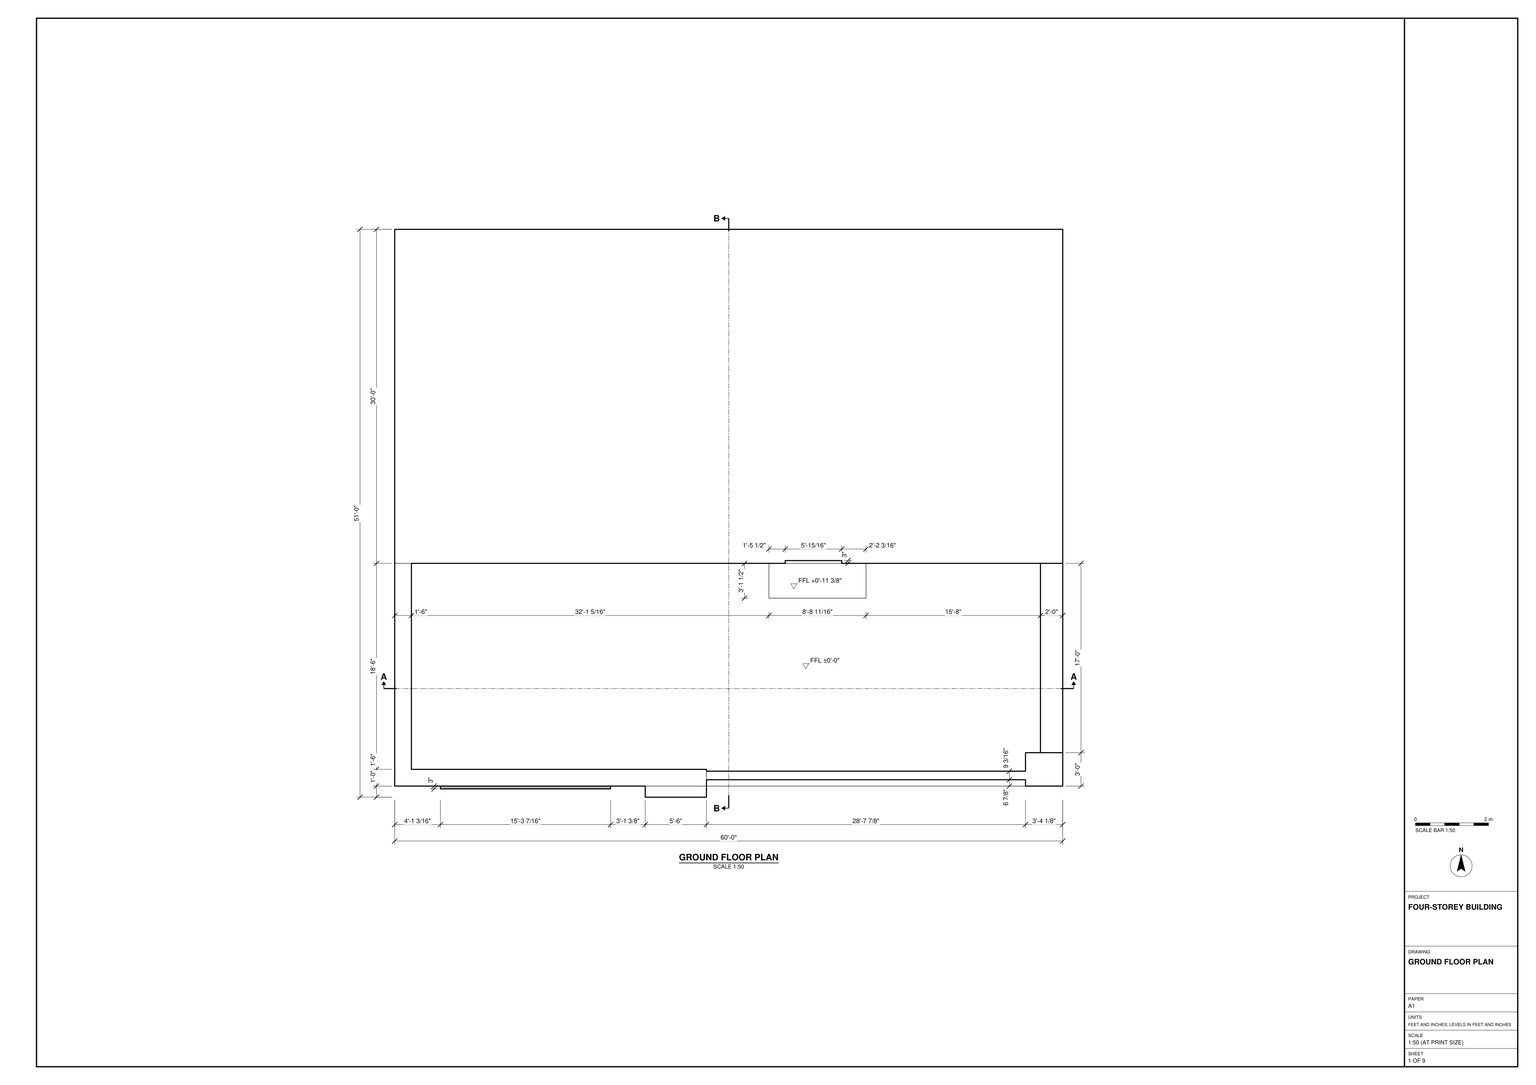
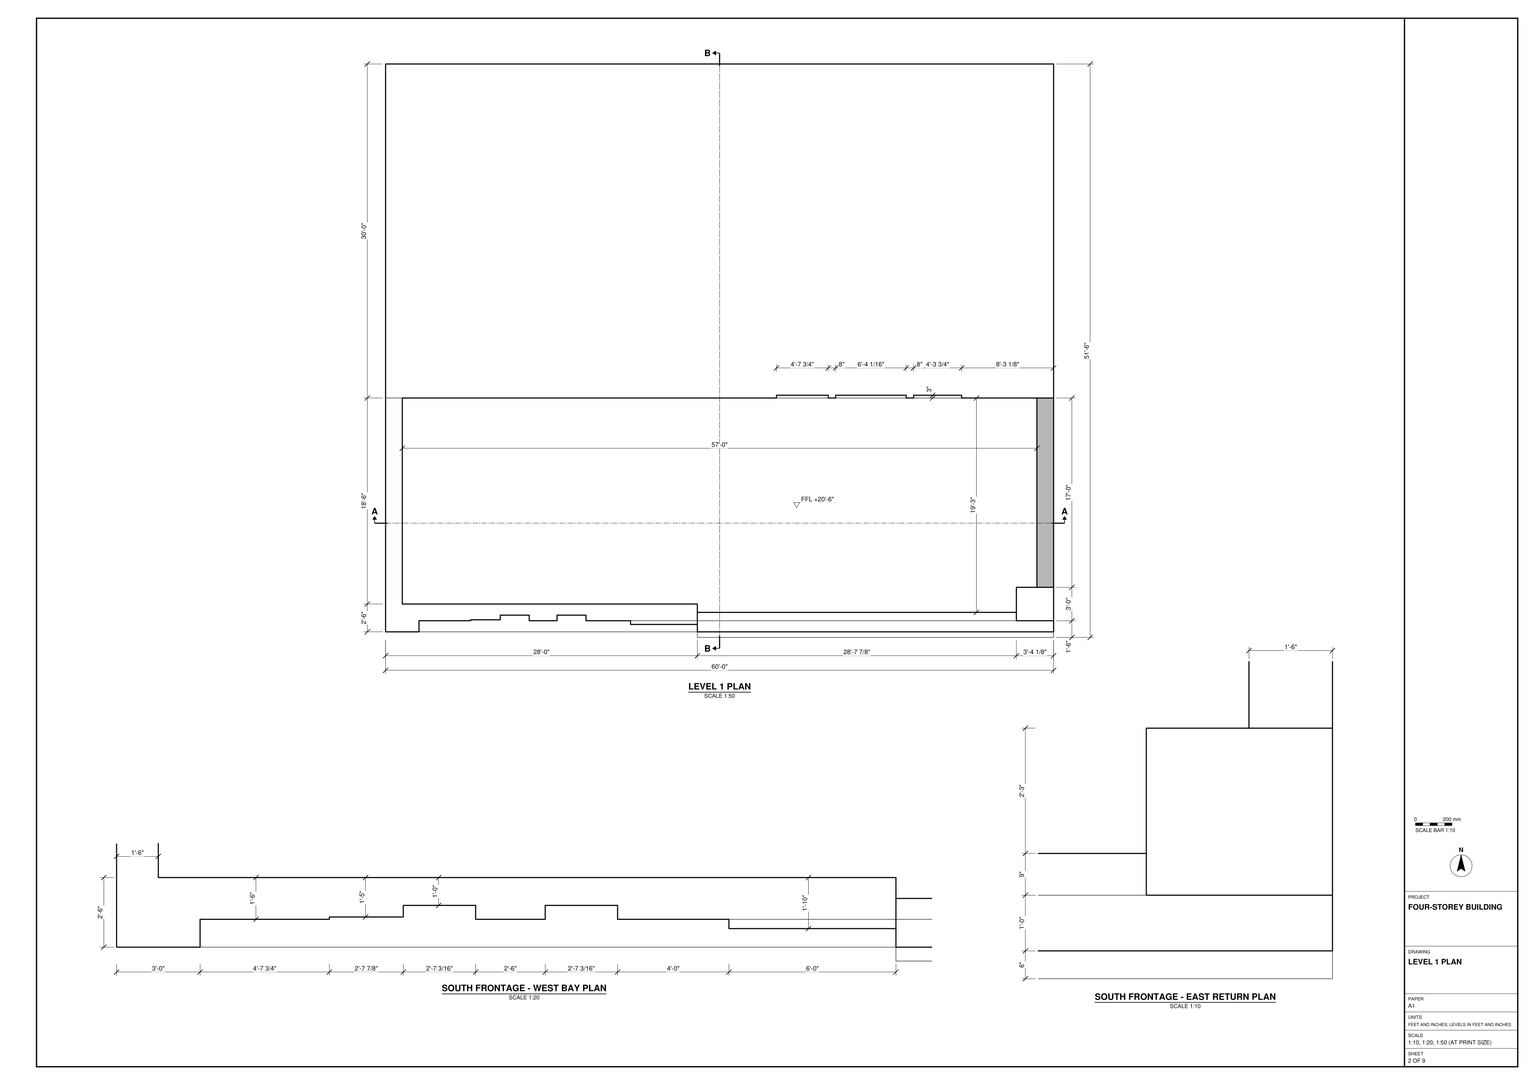
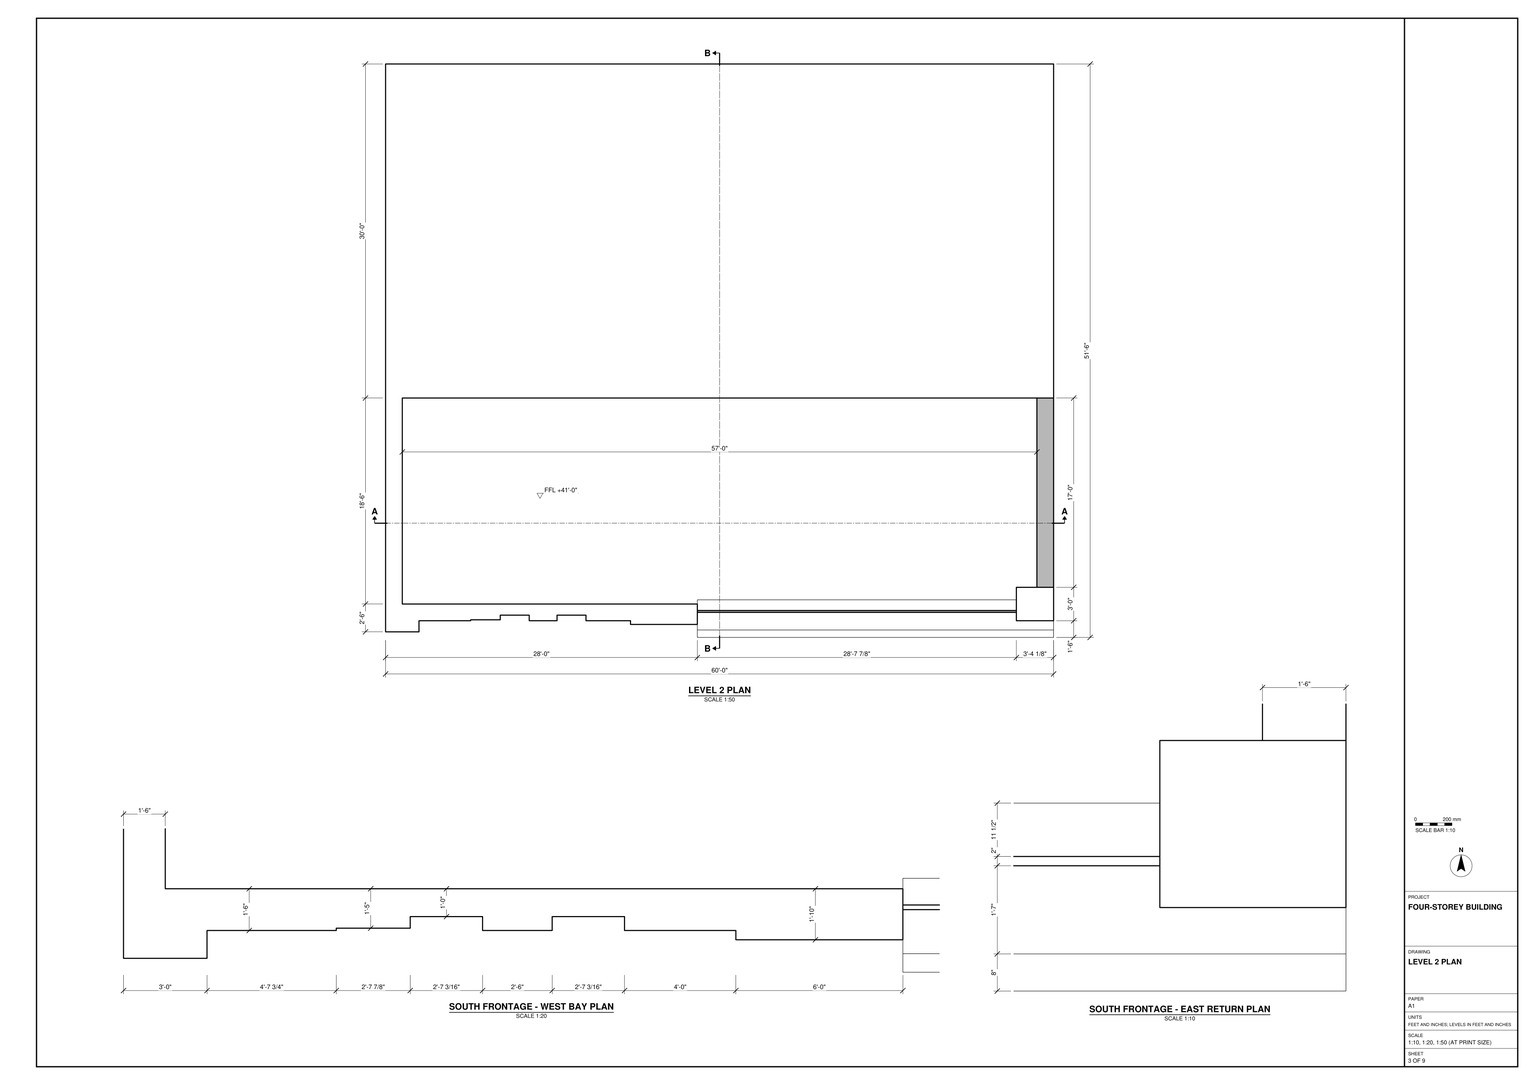
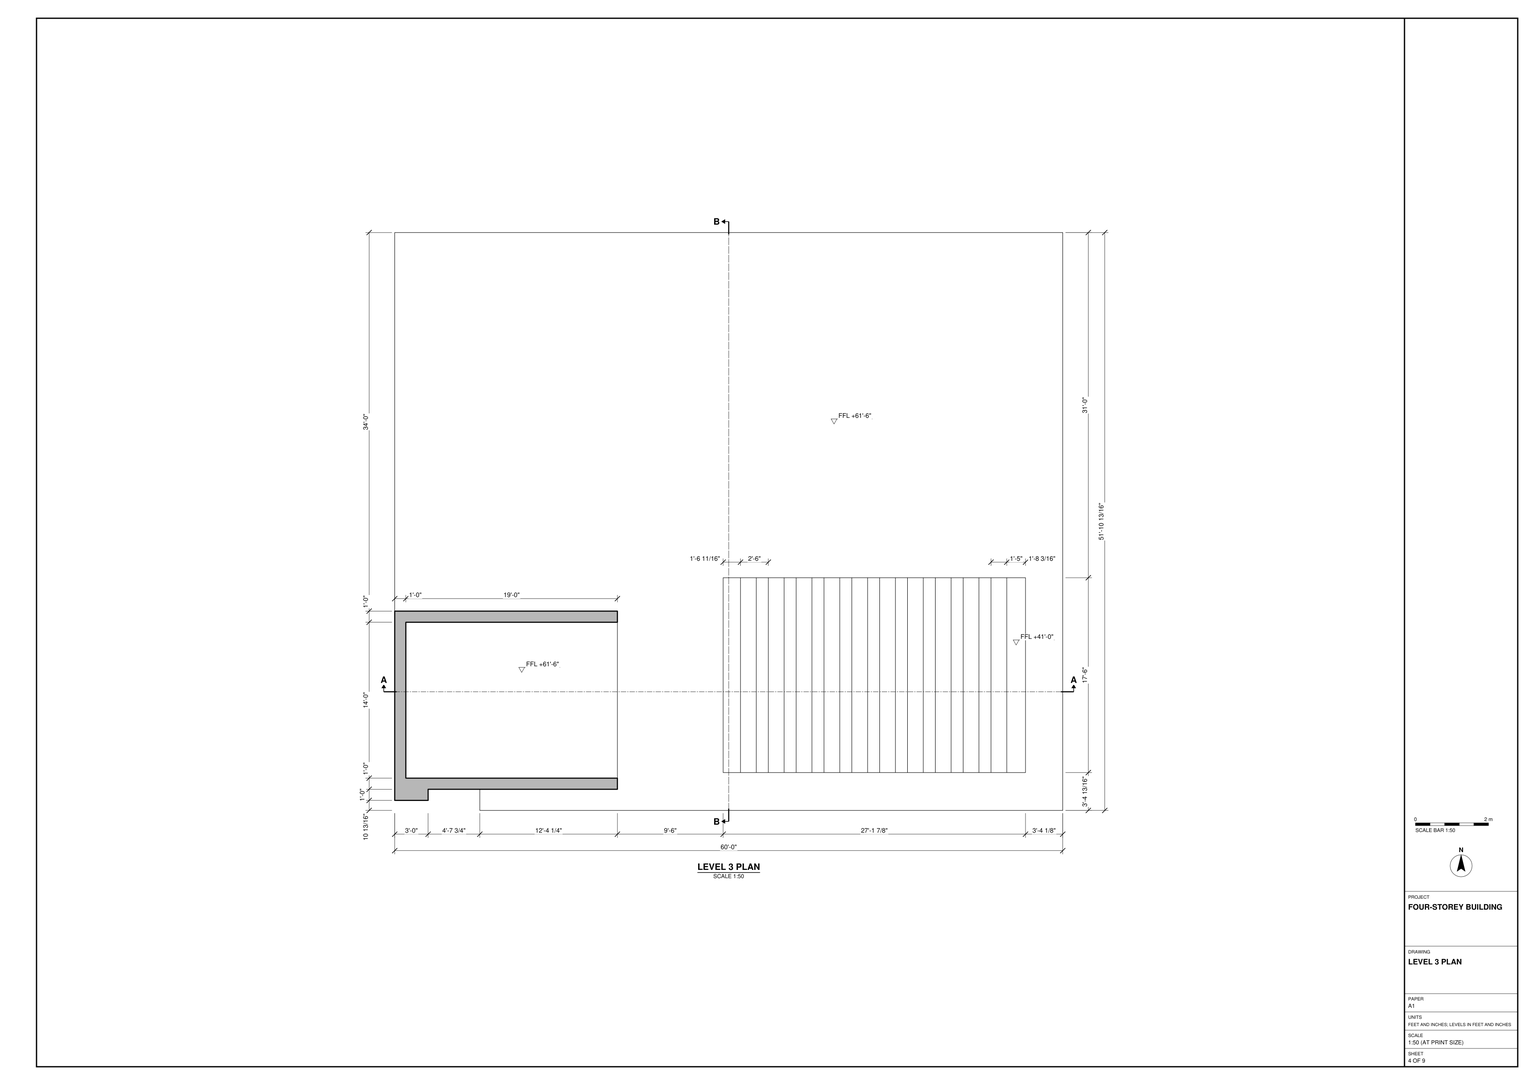
Build the four-storey building in SketchUp using task_files/diagram_01.pdf. Work in feet and inches. The overall dimensions are 60'-0" east to west, 51'-10 13/16" north to south and 70'-0" high. Set the finished floor levels to ±0'-0", +20'-6", +41'-0" and +61'-6".

Lay out the full-width rectangular northern portion first, then use the plan for each floor to form the south frontage. At ground level, include the raised rectangular area east of centre and the projections along the south edge. For levels 1 and 2, use the enlarged west bay plans to set out the changes in depth. Follow the east return details for each level rather than copying the same profile to both. Model the wall thicknesses, openings, floor slabs and roof profile as drawn. Include stairs, built-in joinery and main furniture only where the sheets show them.

Keep walls, slabs and roof elements in separate groups or components. Keep each furniture or joinery piece separate and use components for repeated parts. Any decor or loose items shown may be suitable library components. Save one SketchUp model as output_files/four_storey_building_with_a_stepped_south_frontage.skp.

# SketchUp Ruby script. Lengths in inches.
U = 1.inch
M = Sketchup.active_model
def pt(a) = Geom::Point3d.new(a.map { |v| v * U })
def face(e, loops, mat)
  f = e.add_face(loops[0].map { |a| pt(a) })
  loops[1..].each { |l| e.add_face(l.map { |a| pt(a) }).erase! }
  f.material = f.back_material = mat if mat
  f
end
# faces: each face lists its corners as indices into pts; further lists are holes
def faces(e, pts, list, mat = nil) = list.each { |f| face(e, (f[0].is_a?(Array) ? f : [f]).map { |l| l.map { |i| pts[i] } }, mat) }
# xy, xz, yz: faces in a plane at the given z, y or x. An outline is a flat list of corners, or four numbers for a rectangle; further outlines are holes
def ring(l) = l.size == 4 ? [[l[0], l[1]], [l[2], l[1]], [l[2], l[3]], [l[0], l[3]]] : l.each_slice(2).to_a
def flat(e, list, mat, &to3) = list.each { |f| face(e, (f[0].is_a?(Array) ? f : [f]).map { |l| ring(l).map { |u, v| to3.(u, v) } }, mat) }
def xy(e, z, list, mat = nil) = flat(e, list, mat) { |x, y| [x, y, z] }
def xz(e, y, list, mat = nil) = flat(e, list, mat) { |x, z| [x, y, z] }
def yz(e, x, list, mat = nil) = flat(e, list, mat) { |y, z| [x, y, z] }
def lines(e, pts, list) = list.each { |a, b| e.add_line(pt(pts[a]), pt(pts[b])) }
# prism: a flat outline (further loops are holes) pulled along v
def prism(e, loops, v, mat = nil)
  f = face(e, loops, mat); d = Geom::Vector3d.new(v.map { |x| x * U })
  f.pushpull(f.normal.samedirection?(d) ? d.length : -d.length)
end
def box(e, o, s, mat = nil) = prism(e, [[o, [o[0] + s[0], o[1], o[2]], [o[0] + s[0], o[1] + s[1], o[2]], [o[0], o[1] + s[1], o[2]]]], [0, 0, s[2]], mat)
def at(x, y, z, deg = 0) = Geom::Transformation.translation(pt([x, y, z])) * Geom::Transformation.rotation(ORIGIN, Z_AXIS, deg.degrees)
def axes(o, x, y, z) = Geom::Transformation.new([*x, 0, *y, 0, *z, 0, *pt(o).to_a, 1])
def part(name) = M.definitions.add(name)
# library, detail: a bought-in or finely detailed component or shape, given as its bounding box
def library(name, o, s) = part(name).tap { |d| box(d.entities, o, s) }
def detail(e, o, s) = box(e.add_group.entities, o, s)
def put(e, d, t, mat = nil) = e.add_instance(d, t).tap { |i| i.material = mat if mat }
def group(e, t, mat = nil) = e.add_group.tap { |g| g.transformation = t; g.material = mat if mat }.entities
root = M.entities
M.materials.add("[0110_LightSlateGray]").color = [119, 136, 153]
M.materials.add("[0111_SlateGray]").color = [61, 70, 79]
M.materials.add("[0116_Lavender]").color = [187, 187, 204]
M.materials.add("[0118_Thistle]").color = [216, 191, 216]
M.materials.add("[0119_RosyBrown]").color = [188, 143, 143]
M.materials.add("[0135_DarkGray]").color = [81, 81, 81]
M.materials.add("[0136_Charcoal]").color = [30, 30, 30]
M.materials.add("[0137_Black]").color = [0, 0, 0]
M.materials.add("[Beadboard]").color = [168, 110, 69]
M.materials.add("[Blacktop New]").color = [30, 30, 30]
M.materials.add("[Carrera Marble]").color = [160, 160, 160]
M.materials.add("[Granite Dark Gray]").color = [69, 68, 68]
M.materials.add("[Stone Vein Gray]").color = [166, 165, 165]
M.materials.add("[Translucent Glass Blue]").color = [100, 149, 237]
M.materials["[Translucent Glass Blue]"].alpha = 0.5
M.materials.add("[Translucent Glass Gray]").color = [128, 128, 128]
M.materials["[Translucent Glass Gray]"].alpha = 0.5
xy(root,0,[[0,22.8,720,622.8]])
xy(root,6,[[270,10.8,336,22.8],[0,22.8,0,262.8,18,262.8,18,40.8,336,40.8,336,22.8],[679.875,22.8,679.875,29.65,336,29.65,336,38.84,679.875,38.84,679.875,58.8,720,58.8,720,22.8],[696,58.8,720,262.8],[403.31,225.3,508,262.8],
  [0,262.8,720,622.8]])
xy(root,6,[[336,22.8,679.875,29.65],[336,38.84,679.875,38.84,679.875,58.8,696,58.8,696,262.8,508,262.8,508,225.3,403.31,225.3,403.31,262.8,18,262.8,18,40.8,336,40.8]],"[Granite Dark Gray]")
xy(root,17.375,[[403.31,225.3,508,262.8]],"[Granite Dark Gray]")
xy(root,28.97,[[420.85,262.8,481.8,265.8]])
xy(root,30.43,[[49.22,19.8,232.64,22.8]])
xy(root,102,[[696,58.8,720,262.8]])
xy(root,114.91,[[610.12,262.8,640.875,265.8]])
xy(root,146.85,[[49.22,19.8,232.64,22.8]])
xy(root,152.5,[[336,29.65,679.875,38.84]],"[0137_Black]")
xy(root,180,[[0,10.8,270,22.8]])
xy(root,195.05,[[420.85,262.8,481.8,265.8]])
xy(root,197.24,[[610.12,262.8,640.875,265.8]])
xy(root,246,[[264,18.8,336,22.8],[381.67,35.71,380.14,36.06,378.76,36.79,377.61,37.85,376.77,39.18,376.31,40.67,376.24,42.24,376.59,43.76,377.32,45.15,378.38,46.3,379.71,47.14,381.2,47.6,382.77,47.66,384.29,47.32,385.68,46.59,386.83,45.53,387.67,44.2,388.13,42.71,388.19,41.14,387.85,39.61,387.12,38.23,386.06,37.08,384.73,36.24,383.24,35.78],[464.17,35.71,462.64,36.06,461.26,36.79,460.11,37.85,459.27,39.18,458.81,40.67,458.74,42.24,459.09,43.76,459.82,45.15,460.88,46.3,462.21,47.14,463.7,47.6,465.27,47.66,466.79,47.32,468.18,46.59,469.33,45.53,470.17,44.2,470.63,42.71,470.69,41.14,470.35,39.61,469.62,38.23,468.56,37.08,467.23,36.24,465.74,35.78],[571.98,35.71,570.46,36.06,569.07,36.79,567.92,37.85,567.08,39.18,566.62,40.67,566.56,42.24,566.9,43.76,567.63,45.15,568.69,46.3,570.02,47.14,571.51,47.6,573.08,47.66,574.61,47.32,575.99,46.59,577.14,45.53,577.98,44.2,578.44,42.71,578.51,41.14,578.16,39.61,577.43,38.23,576.37,37.08,575.04,36.24,573.55,35.78],[638.55,35.71,637.02,36.06,635.63,36.79,634.48,37.85,633.65,39.18,633.18,40.67,633.12,42.24,633.46,43.76,634.19,45.15,635.26,46.3,636.58,47.14,638.08,47.6,639.64,47.66,641.17,47.32,642.56,46.59,643.71,45.53,644.54,44.2,645.01,42.71,645.07,41.14,644.72,39.61,643.99,38.23,642.93,37.08,641.61,36.24,640.11,35.78],
  [400.99,114.11,399.46,114.46,398.08,115.1875,396.93,116.25,396.09,117.57,395.625,119.07,395.5625,120.63,395.91,122.16,396.64,123.55,397.7,124.7,399.03,125.54,400.52,126,402.09,126.0625,403.61,125.72,405,124.99,406.15,123.92,406.99,122.6,407.45,121.1,407.51,119.54,407.17,118.01,406.4375,116.625,405.375,115.48,404.05,114.64,402.56,114.17],[503.93,114.11,502.4,114.46,501.01,115.1875,499.86,116.25,499.03,117.57,498.5625,119.07,498.5,120.63,498.85,122.16,499.58,123.55,500.64,124.7,501.96,125.54,503.46,126,505.02,126.0625,506.55,125.72,507.9375,124.99,509.09,123.92,509.92,122.6,510.39,121.1,510.45,119.54,510.11,118.01,509.375,116.625,508.3125,115.48,506.99,114.64,505.49,114.17],[620.87,114.11,619.34,114.46,617.95,115.1875,616.8,116.25,615.97,117.57,615.5,119.07,615.4375,120.63,615.78,122.16,616.51,123.55,617.58,124.7,618.9,125.54,620.4,126,621.96,126.0625,623.49,125.72,624.875,124.99,626.03,123.92,626.86,122.6,627.33,121.1,627.39,119.54,627.04,118.01,626.3125,116.625,625.25,115.48,623.93,114.64,622.43,114.17]])
xy(root,246,[[36,10.8,336,10.8,336,18.8,264,18.8,264,22.8,216,22.8,216,28.8,184.8,28.8,184.8,22.8,154.8,22.8,154.8,28.8,123.6,28.8,123.6,23.8,91.72,23.8,91.72,22.8,36,22.8]],"[0111_SlateGray]")
xy(root,246,[[[336,4.8,336,40.8,18,40.8,18,262.8,720,262.8,720,58.8,679.875,58.8,679.875,22.8,720,22.8,720,4.8],[400.99,114.11,402.56,114.17,404.05,114.64,405.375,115.48,406.4375,116.625,407.17,118.01,407.51,119.54,407.45,121.1,406.99,122.6,406.15,123.92,405,124.99,403.61,125.72,402.09,126.0625,400.52,126,399.03,125.54,397.7,124.7,396.64,123.55,395.91,122.16,395.5625,120.63,395.625,119.07,396.09,117.57,396.93,116.25,398.08,115.1875,399.46,114.46],[503.93,114.11,505.49,114.17,506.99,114.64,508.3125,115.48,509.375,116.625,510.11,118.01,510.45,119.54,510.39,121.1,509.92,122.6,509.09,123.92,507.9375,124.99,506.55,125.72,505.02,126.0625,503.46,126,501.96,125.54,500.64,124.7,499.58,123.55,498.85,122.16,498.5,120.63,498.5625,119.07,499.03,117.57,499.86,116.25,501.01,115.1875,502.4,114.46],[620.87,114.11,622.43,114.17,623.93,114.64,625.25,115.48,626.3125,116.625,627.04,118.01,627.39,119.54,627.33,121.1,626.86,122.6,626.03,123.92,624.875,124.99,623.49,125.72,621.96,126.0625,620.4,126,618.9,125.54,617.58,124.7,616.51,123.55,615.78,122.16,615.4375,120.63,615.5,119.07,615.97,117.57,616.8,116.25,617.95,115.1875,619.34,114.46],[381.67,35.71,383.24,35.78,384.73,36.24,386.06,37.08,387.12,38.23,387.85,39.61,388.19,41.14,388.13,42.71,387.67,44.2,386.83,45.53,385.68,46.59,384.29,47.32,382.77,47.66,381.2,47.6,379.71,47.14,378.38,46.3,377.32,45.15,376.59,43.76,376.24,42.24,376.31,40.67,376.77,39.18,377.61,37.85,378.76,36.79,380.14,36.06],[638.55,35.71,640.11,35.78,641.61,36.24,642.93,37.08,643.99,38.23,644.72,39.61,645.07,41.14,645.01,42.71,644.54,44.2,643.71,45.53,642.56,46.59,641.17,47.32,639.64,47.66,638.08,47.6,636.58,47.14,635.26,46.3,634.19,45.15,633.46,43.76,633.12,42.24,633.18,40.67,633.65,39.18,634.48,37.85,635.63,36.79,637.02,36.06],[571.98,35.71,573.55,35.78,575.04,36.24,576.37,37.08,577.43,38.23,578.16,39.61,578.51,41.14,578.44,42.71,577.98,44.2,577.14,45.53,575.99,46.59,574.61,47.32,573.08,47.66,571.51,47.6,570.02,47.14,568.69,46.3,567.63,45.15,566.9,43.76,566.56,42.24,566.62,40.67,567.08,39.18,567.92,37.85,569.07,36.79,570.46,36.06],[464.17,35.71,465.74,35.78,467.23,36.24,468.56,37.08,469.62,38.23,470.35,39.61,470.69,41.14,470.63,42.71,470.17,44.2,469.33,45.53,468.18,46.59,466.79,47.32,465.27,47.66,463.7,47.6,462.21,47.14,460.88,46.3,459.82,45.15,459.09,43.76,458.74,42.24,458.81,40.67,459.27,39.18,460.11,37.85,461.26,36.79,462.64,36.06]]],"[0119_RosyBrown]")
xy(root,252,[[336,22.8,679.875,31.8],[679.875,22.8,720,58.8],[702,58.8,720,262.8]])
xy(root,252,[[336,31.8,679.875,31.8,679.875,58.8,702,58.8,702,262.8,18,262.8,18,40.8,336,40.8]],"[Carrera Marble]")
xy(root,261,[[336,4.8,720,10.8]])
xy(root,292.66,[[421.33,262.8,477.07,265.8],[485.07,262.8,561.11,265.8],[569.11,262.8,620.86,265.8]])
xy(root,336,[[336,10.8,720,10.8,720,22.8,679.875,22.8,679.875,31.8,336,31.8]],"[0116_Lavender]")
xy(root,348,[[702,58.8,720,262.8]])
xy(root,448.01,[[421.33,262.8,477.07,265.8],[485.07,262.8,561.11,265.8],[569.11,262.8,620.86,265.8]])
xy(root,492,[[375.3,76.82,373.75,77.06,372.3125,77.6875,371.09,78.67,370.17,79.93,369.6,81.39,369.43,82.95,369.66,84.49,370.29,85.93,371.27,87.15,372.54,88.08,374,88.65,375.55,88.82,377.1,88.58,378.53,87.95,379.76,86.97,380.68,85.71,381.25,84.25,381.42,82.69,381.19,81.14,380.56,79.71,379.58,78.49,378.3125,77.56,376.85,76.99],[495.86,76.82,494.31,77.06,492.875,77.6875,491.65,78.67,490.73,79.93,490.16,81.39,489.99,82.95,490.23,84.49,490.86,85.93,491.84,87.15,493.1,88.08,494.56,88.65,496.11,88.82,497.66,88.58,499.1,87.95,500.32,86.97,501.25,85.71,501.8125,84.25,501.99,82.69,501.75,81.14,501.12,79.71,500.14,78.49,498.875,77.56,497.42,76.99],[622.42,76.82,620.87,77.06,619.4375,77.6875,618.22,78.67,617.29,79.93,616.72,81.39,616.55,82.95,616.79,84.49,617.42,85.93,618.4,87.15,619.66,88.08,621.12,88.65,622.68,88.82,624.23,88.58,625.66,87.95,626.88,86.97,627.81,85.71,628.375,84.25,628.55,82.69,628.31,81.14,627.68,79.71,626.7,78.49,625.4375,77.56,623.98,76.99],[427.95,164.04,426.4,164.28,424.97,164.91,423.75,165.89,422.82,167.15,422.25,168.61,422.08,170.17,422.32,171.72,422.95,173.15,423.93,174.37,425.19,175.3,426.65,175.87,428.21,176.04,429.76,175.8,431.19,175.17,432.41,174.19,433.34,172.93,433.91,171.47,434.08,169.91,433.84,168.36,433.21,166.93,432.23,165.71,430.97,164.78,429.51,164.21],[570.27,164.04,568.72,164.28,567.28,164.91,566.0625,165.89,565.13,167.15,564.57,168.61,564.39,170.17,564.63,171.72,565.26,173.15,566.24,174.37,567.5,175.3,568.96,175.87,570.52,176.04,572.07,175.8,573.5,175.17,574.73,174.19,575.65,172.93,576.22,171.47,576.39,169.91,576.15,168.36,575.52,166.93,574.54,165.71,573.28,164.78,571.82,164.21]])
xy(root,492,[[[336,4.8,336,40.8,18,40.8,18,262.8,720,262.8,720,58.8,679.875,58.8,679.875,22.8,720,22.8,720,4.8],[570.27,164.04,571.82,164.21,573.28,164.78,574.54,165.71,575.52,166.93,576.15,168.36,576.39,169.91,576.22,171.47,575.65,172.93,574.73,174.19,573.5,175.17,572.07,175.8,570.52,176.04,568.96,175.87,567.5,175.3,566.24,174.37,565.26,173.15,564.63,171.72,564.39,170.17,564.57,168.61,565.13,167.15,566.0625,165.89,567.28,164.91,568.72,164.28],[427.95,164.04,429.51,164.21,430.97,164.78,432.23,165.71,433.21,166.93,433.84,168.36,434.08,169.91,433.91,171.47,433.34,172.93,432.41,174.19,431.19,175.17,429.76,175.8,428.21,176.04,426.65,175.87,425.19,175.3,423.93,174.37,422.95,173.15,422.32,171.72,422.08,170.17,422.25,168.61,422.82,167.15,423.75,165.89,424.97,164.91,426.4,164.28],[375.3,76.82,376.85,76.99,378.3125,77.56,379.58,78.49,380.56,79.71,381.19,81.14,381.42,82.69,381.25,84.25,380.68,85.71,379.76,86.97,378.53,87.95,377.1,88.58,375.55,88.82,374,88.65,372.54,88.08,371.27,87.15,370.29,85.93,369.66,84.49,369.43,82.95,369.6,81.39,370.17,79.93,371.09,78.67,372.3125,77.6875,373.75,77.06],[495.86,76.82,497.42,76.99,498.875,77.56,500.14,78.49,501.12,79.71,501.75,81.14,501.99,82.69,501.8125,84.25,501.25,85.71,500.32,86.97,499.1,87.95,497.66,88.58,496.11,88.82,494.56,88.65,493.1,88.08,491.84,87.15,490.86,85.93,490.23,84.49,489.99,82.95,490.16,81.39,490.73,79.93,491.65,78.67,492.875,77.6875,494.31,77.06],[622.42,76.82,623.98,76.99,625.4375,77.56,626.7,78.49,627.68,79.71,628.31,81.14,628.55,82.69,628.375,84.25,627.81,85.71,626.88,86.97,625.66,87.95,624.23,88.58,622.68,88.82,621.12,88.65,619.66,88.08,618.4,87.15,617.42,85.93,616.79,84.49,616.55,82.95,616.72,81.39,617.29,79.93,618.22,78.67,619.4375,77.6875,620.87,77.06]]],"[0119_RosyBrown]")
xy(root,498,[[336,4.8,720,12.8],[336,12.8,336,31.8,679.875,31.8,679.875,22.8,720,22.8,720,12.8],[679.875,22.8,720,58.8],[336,31.8,679.875,45.3],[702,58.8,720,262.8]])
xy(root,498,[[18,40.8,336,40.8,336,45.3,679.875,45.3,679.875,58.8,702,58.8,702,262.8,18,262.8]],"[Carrera Marble]")
xy(root,534,[[336,31.8,679.875,33.8],[336,33.8,679.875,45.3]])
xy(root,534,[[336,12.8,720,12.8,720,22.8,679.875,22.8,679.875,31.8,336,31.8]],"[Blacktop New]")
xy(root,556.15,[[419.07,262.8,477.07,265.8],[485.07,262.8,561.11,265.8],[569.11,262.8,623.11,265.8]])
xy(root,594,[[702,58.8,720,262.8]])
xy(root,597,[[336,31.8,679.875,33.8]])
xy(root,690.375,[[419.07,262.8,477.07,265.8],[485.07,262.8,561.11,265.8],[569.11,262.8,623.11,265.8]])
xy(root,720,[[[91.72,0,91.72,22.8,123.6,22.8,123.6,28.8,154.8,28.8,154.8,22.8,184.8,22.8,184.8,28.8,216,28.8,216,22.8,264,22.8,264,18.8,336,18.8,336,40.8,679.875,40.8,679.875,22.8,720,22.8,720,0],[194.31,7.2,195.83,7.6,197.1875,8.37,198.3,9.47,199.1,10.82,199.51,12.33,199.53,13.89,199.13,15.41,198.36,16.77,197.26,17.89,195.91,18.68,194.4,19.1,192.83,19.11,191.32,18.72,189.96,17.94,188.84,16.84,188.05,15.49,187.63,13.98,187.62,12.42,188.01,10.9,188.78,9.54,189.88,8.42,191.23,7.63,192.74,7.21],[249.43,7.2,250.95,7.6,252.3125,8.37,253.43,9.47,254.22,10.82,254.64,12.33,254.65,13.89,254.26,15.41,253.49,16.77,252.39,17.89,251.04,18.68,249.53,19.1,247.96,19.11,246.44,18.72,245.08,17.94,243.97,16.84,243.17,15.49,242.75,13.98,242.74,12.42,243.14,10.9,243.91,9.54,245.01,8.42,246.36,7.63,247.87,7.21],[359.5,7.2,361.01,7.6,362.375,8.37,363.49,9.47,364.29,10.82,364.7,12.33,364.71,13.89,364.32,15.41,363.55,16.77,362.45,17.89,361.1,18.68,359.59,19.1,358.02,19.11,356.51,18.72,355.14,17.94,354.03,16.84,353.23,15.49,352.82,13.98,352.81,12.42,353.2,10.9,353.97,9.54,355.07,8.42,356.42,7.63,357.93,7.21],[430.06,7.2,431.58,7.6,432.9375,8.37,434.05,9.47,434.85,10.82,435.26,12.33,435.28,13.89,434.88,15.41,434.11,16.77,433.01,17.89,431.66,18.68,430.15,19.1,428.58,19.11,427.07,18.72,425.71,17.94,424.59,16.84,423.8,15.49,423.38,13.98,423.37,12.42,423.76,10.9,424.53,9.54,425.63,8.42,426.98,7.63,428.49,7.21],[498.31,7.2,499.83,7.6,501.1875,8.37,502.3,9.47,503.1,10.82,503.51,12.33,503.53,13.89,503.13,15.41,502.36,16.77,501.26,17.89,499.91,18.68,498.4,19.1,496.83,19.11,495.32,18.72,493.96,17.94,492.84,16.84,492.05,15.49,491.63,13.98,491.62,12.42,492.01,10.9,492.78,9.54,493.88,8.42,495.23,7.63,496.74,7.21],[570.43,7.2,571.95,7.6,573.3125,8.37,574.43,9.47,575.22,10.82,575.64,12.33,575.65,13.89,575.26,15.41,574.49,16.77,573.39,17.89,572.04,18.68,570.53,19.1,568.96,19.11,567.44,18.72,566.08,17.94,564.97,16.84,564.17,15.49,563.75,13.98,563.74,12.42,564.14,10.9,564.91,9.54,566.01,8.42,567.36,7.63,568.87,7.21],[643.25,7.2,644.76,7.6,646.125,8.37,647.24,9.47,648.04,10.82,648.45,12.33,648.46,13.89,648.07,15.41,647.3,16.77,646.2,17.89,644.85,18.68,643.34,19.1,641.77,19.11,640.26,18.72,638.89,17.94,637.78,16.84,636.98,15.49,636.57,13.98,636.56,12.42,636.95,10.9,637.72,9.54,638.82,8.42,640.17,7.63,641.68,7.21],[302.91,3.78,304.43,4.17,305.79,4.95,306.91,6.04,307.7,7.4,308.12,8.9,308.13,10.47,307.74,11.99,306.96,13.35,305.86,14.47,304.51,15.26,303,15.68,301.4375,15.6875,299.92,15.29,298.56,14.52,297.44,13.42,296.65,12.07,296.23,10.5625,296.22,9,296.61,7.48,297.39,6.12,298.49,5,299.84,4.21,301.35,3.79],[141.18,7.2,142.7,7.6,144.0625,8.37,145.18,9.47,145.97,10.82,146.39,12.33,146.4,13.89,146.01,15.41,145.24,16.77,144.14,17.89,142.79,18.68,141.28,19.1,139.71,19.11,138.19,18.72,136.83,17.94,135.72,16.84,134.92,15.49,134.5,13.98,134.49,12.42,134.89,10.9,135.66,9.54,136.76,8.42,138.11,7.63,139.62,7.21]],[302.91,3.78,301.35,3.79,299.84,4.21,298.49,5,297.39,6.12,296.61,7.48,296.22,9,296.23,10.5625,296.65,12.07,297.44,13.42,298.56,14.52,299.92,15.29,301.4375,15.6875,303,15.68,304.51,15.26,305.86,14.47,306.96,13.35,307.74,11.99,308.13,10.47,308.12,8.9,307.7,7.4,306.91,6.04,305.79,4.95,304.43,4.17],[141.18,7.2,139.62,7.21,138.11,7.63,136.76,8.42,135.66,9.54,134.89,10.9,134.49,12.42,134.5,13.98,134.92,15.49,135.72,16.84,136.83,17.94,138.19,18.72,139.71,19.11,141.28,19.1,142.79,18.68,144.14,17.89,145.24,16.77,146.01,15.41,146.4,13.89,146.39,12.33,145.97,10.82,145.18,9.47,144.0625,8.37,142.7,7.6],[194.31,7.2,192.74,7.21,191.23,7.63,189.88,8.42,188.78,9.54,188.01,10.9,187.62,12.42,187.63,13.98,188.05,15.49,188.84,16.84,189.96,17.94,191.32,18.72,192.83,19.11,194.4,19.1,195.91,18.68,197.26,17.89,198.36,16.77,199.13,15.41,199.53,13.89,199.51,12.33,199.1,10.82,198.3,9.47,197.1875,8.37,195.83,7.6],[249.43,7.2,247.87,7.21,246.36,7.63,245.01,8.42,243.91,9.54,243.14,10.9,242.74,12.42,242.75,13.98,243.17,15.49,243.97,16.84,245.08,17.94,246.44,18.72,247.96,19.11,249.53,19.1,251.04,18.68,252.39,17.89,253.49,16.77,254.26,15.41,254.65,13.89,254.64,12.33,254.22,10.82,253.43,9.47,252.3125,8.37,250.95,7.6],
  [359.5,7.2,357.93,7.21,356.42,7.63,355.07,8.42,353.97,9.54,353.2,10.9,352.81,12.42,352.82,13.98,353.23,15.49,354.03,16.84,355.14,17.94,356.51,18.72,358.02,19.11,359.59,19.1,361.1,18.68,362.45,17.89,363.55,16.77,364.32,15.41,364.71,13.89,364.7,12.33,364.29,10.82,363.49,9.47,362.375,8.37,361.01,7.6],[430.06,7.2,428.49,7.21,426.98,7.63,425.63,8.42,424.53,9.54,423.76,10.9,423.37,12.42,423.38,13.98,423.8,15.49,424.59,16.84,425.71,17.94,427.07,18.72,428.58,19.11,430.15,19.1,431.66,18.68,433.01,17.89,434.11,16.77,434.88,15.41,435.28,13.89,435.26,12.33,434.85,10.82,434.05,9.47,432.9375,8.37,431.58,7.6],[498.31,7.2,496.74,7.21,495.23,7.63,493.88,8.42,492.78,9.54,492.01,10.9,491.62,12.42,491.63,13.98,492.05,15.49,492.84,16.84,493.96,17.94,495.32,18.72,496.83,19.11,498.4,19.1,499.91,18.68,501.26,17.89,502.36,16.77,503.13,15.41,503.53,13.89,503.51,12.33,503.1,10.82,502.3,9.47,501.1875,8.37,499.83,7.6],[570.43,7.2,568.87,7.21,567.36,7.63,566.01,8.42,564.91,9.54,564.14,10.9,563.74,12.42,563.75,13.98,564.17,15.49,564.97,16.84,566.08,17.94,567.44,18.72,568.96,19.11,570.53,19.1,572.04,18.68,573.39,17.89,574.49,16.77,575.26,15.41,575.65,13.89,575.64,12.33,575.22,10.82,574.43,9.47,573.3125,8.37,571.95,7.6],[643.25,7.2,641.68,7.21,640.17,7.63,638.82,8.42,637.72,9.54,636.95,10.9,636.56,12.42,636.57,13.98,636.98,15.49,637.78,16.84,638.89,17.94,640.26,18.72,641.77,19.11,643.34,19.1,644.85,18.68,646.2,17.89,647.3,16.77,648.07,15.41,648.46,13.89,648.45,12.33,648.04,10.82,647.24,9.47,646.125,8.37,644.76,7.6],
  [264,18.8,336,22.8],[91.72,22.8,123.6,23.8],[679.875,22.8,720,58.8],[[336,40.8,336,262.8,720,262.8,720,58.8,679.875,58.8,679.875,250.8,354,250.8,354,40.8],[390.73,254.08,391.51,254.1875,392.23,254.49,392.86,254.96,393.33,255.58,393.63,256.31,393.73,257.08,393.63,257.86,393.33,258.58,392.86,259.21,392.23,259.68,391.51,259.98,390.73,260.08,389.96,259.98,389.23,259.68,388.61,259.21,388.14,258.58,387.84,257.86,387.73,257.08,387.84,256.31,388.14,255.58,388.61,254.96,389.23,254.49,389.96,254.1875],[414.73,254.08,415.51,254.1875,416.23,254.49,416.86,254.96,417.33,255.58,417.63,256.31,417.73,257.08,417.63,257.86,417.33,258.58,416.86,259.21,416.23,259.68,415.51,259.98,414.73,260.08,413.96,259.98,413.23,259.68,412.61,259.21,412.14,258.58,411.84,257.86,411.73,257.08,411.84,256.31,412.14,255.58,412.61,254.96,413.23,254.49,413.96,254.1875],[438.73,254.08,439.51,254.1875,440.23,254.49,440.86,254.96,441.33,255.58,441.63,256.31,441.73,257.08,441.63,257.86,441.33,258.58,440.86,259.21,440.23,259.68,439.51,259.98,438.73,260.08,437.96,259.98,437.23,259.68,436.61,259.21,436.14,258.58,435.84,257.86,435.73,257.08,435.84,256.31,436.14,255.58,436.61,254.96,437.23,254.49,437.96,254.1875],[462.73,254.08,463.51,254.1875,464.23,254.49,464.86,254.96,465.33,255.58,465.63,256.31,465.73,257.08,465.63,257.86,465.33,258.58,464.86,259.21,464.23,259.68,463.51,259.98,462.73,260.08,461.96,259.98,461.23,259.68,460.61,259.21,460.14,258.58,459.84,257.86,459.73,257.08,459.84,256.31,460.14,255.58,460.61,254.96,461.23,254.49,461.96,254.1875],[486.73,254.08,487.51,254.1875,488.23,254.49,488.86,254.96,489.33,255.58,489.63,256.31,489.73,257.08,489.63,257.86,489.33,258.58,488.86,259.21,488.23,259.68,487.51,259.98,486.73,260.08,485.96,259.98,485.23,259.68,484.61,259.21,484.14,258.58,483.84,257.86,483.73,257.08,483.84,256.31,484.14,255.58,484.61,254.96,485.23,254.49,485.96,254.1875],[366.73,254.08,367.51,254.1875,368.23,254.49,368.86,254.96,369.33,255.58,369.63,256.31,369.73,257.08,369.63,257.86,369.33,258.58,368.86,259.21,368.23,259.68,367.51,259.98,366.73,260.08,365.96,259.98,365.23,259.68,364.61,259.21,364.14,258.58,363.84,257.86,363.73,257.08,363.84,256.31,364.14,255.58,364.61,254.96,365.23,254.49,365.96,254.1875]],[366.73,254.08,365.96,254.1875,365.23,254.49,364.61,254.96,364.14,255.58,363.84,256.31,363.73,257.08,363.84,257.86,364.14,258.58,364.61,259.21,365.23,259.68,365.96,259.98,366.73,260.08,367.51,259.98,368.23,259.68,368.86,259.21,369.33,258.58,369.63,257.86,369.73,257.08,369.63,256.31,369.33,255.58,368.86,254.96,368.23,254.49,367.51,254.1875],
  [390.73,254.08,389.96,254.1875,389.23,254.49,388.61,254.96,388.14,255.58,387.84,256.31,387.73,257.08,387.84,257.86,388.14,258.58,388.61,259.21,389.23,259.68,389.96,259.98,390.73,260.08,391.51,259.98,392.23,259.68,392.86,259.21,393.33,258.58,393.63,257.86,393.73,257.08,393.63,256.31,393.33,255.58,392.86,254.96,392.23,254.49,391.51,254.1875],[414.73,254.08,413.96,254.1875,413.23,254.49,412.61,254.96,412.14,255.58,411.84,256.31,411.73,257.08,411.84,257.86,412.14,258.58,412.61,259.21,413.23,259.68,413.96,259.98,414.73,260.08,415.51,259.98,416.23,259.68,416.86,259.21,417.33,258.58,417.63,257.86,417.73,257.08,417.63,256.31,417.33,255.58,416.86,254.96,416.23,254.49,415.51,254.1875],[438.73,254.08,437.96,254.1875,437.23,254.49,436.61,254.96,436.14,255.58,435.84,256.31,435.73,257.08,435.84,257.86,436.14,258.58,436.61,259.21,437.23,259.68,437.96,259.98,438.73,260.08,439.51,259.98,440.23,259.68,440.86,259.21,441.33,258.58,441.63,257.86,441.73,257.08,441.63,256.31,441.33,255.58,440.86,254.96,440.23,254.49,439.51,254.1875],[462.73,254.08,461.96,254.1875,461.23,254.49,460.61,254.96,460.14,255.58,459.84,256.31,459.73,257.08,459.84,257.86,460.14,258.58,460.61,259.21,461.23,259.68,461.96,259.98,462.73,260.08,463.51,259.98,464.23,259.68,464.86,259.21,465.33,258.58,465.63,257.86,465.73,257.08,465.63,256.31,465.33,255.58,464.86,254.96,464.23,254.49,463.51,254.1875],[486.73,254.08,485.96,254.1875,485.23,254.49,484.61,254.96,484.14,255.58,483.84,256.31,483.73,257.08,483.84,257.86,484.14,258.58,484.61,259.21,485.23,259.68,485.96,259.98,486.73,260.08,487.51,259.98,488.23,259.68,488.86,259.21,489.33,258.58,489.63,257.86,489.73,257.08,489.63,256.31,489.33,255.58,488.86,254.96,488.23,254.49,487.51,254.1875]])
xy(root,726.9375,[[372.68,40.8,389.68,250.8],[402.68,40.8,419.68,250.8],[432.68,40.8,449.68,250.8],[462.68,40.8,479.68,250.8],[492.68,40.8,509.68,250.8],
  [522.68,40.8,539.68,250.8],[552.68,40.8,569.68,250.8],[582.68,40.8,599.68,250.8],[612.68,40.8,629.68,250.8],[642.68,40.8,659.68,250.8]],"[0136_Charcoal]")
xy(root,738,[[18,40.8,336,262.8]])
xy(root,739.1875,[[372.68,40.8,389.68,250.8],[402.68,40.8,419.68,250.8],[432.68,40.8,449.68,250.8],[462.68,40.8,479.68,250.8],[492.68,40.8,509.68,250.8],
  [522.68,40.8,539.68,250.8],[552.68,40.8,569.68,250.8],[582.68,40.8,599.68,250.8],[612.68,40.8,629.68,250.8],[642.68,40.8,659.68,250.8]],"[0136_Charcoal]")
xy(root,744,[[[91.72,0,720,0,720,622.8,0,622.8,0,214.8,240,214.8,240,22.8,91.72,22.8],[354,40.8,679.875,250.8]],[123.42,22.8,153.92,28.8],[184.8,22.8,215.3,28.8],[12,34.8,240,202.8]])
xy(root,779.5,[[123.42,22.8,153.92,28.8],[184.8,22.8,215.3,28.8]])
xy(root,810,[[36,10.8,240,22.8]],"[0111_SlateGray]")
xy(root,828,[[12,34.8,240,37.17],[12,37.17,240,202.8]])
xy(root,840,[[0,10.8,240,10.8,240,34.8,12,34.8,12,202.8,240,202.8,240,214.8,0,214.8],[12,34.8,240,202.8]],"[0111_SlateGray]")
xz(root,0,[[91.72,720,720,744]])
xz(root,4.8,[[336,246,720,261],[336,492,720,498]])
xz(root,10.8,[[270,6,336,6,336,246,36,246,36,810,240,810,240,840,0,840,0,180,270,180]],"[0111_SlateGray]")
xz(root,10.8,[[336,261,720,336]],"[0116_Lavender]")
xz(root,12.8,[[336,498,720,534]],"[Blacktop New]")
xz(root,18.8,[[264,246,336,720]],"[Stone Vein Gray]")
xz(root,19.8,[[49.22,30.43,232.64,146.85]],"[0118_Thistle]")
xz(root,22.8,[[[37.24,18.45,244.62,158.83],[49.22,30.43,232.64,146.85]],[49.22,30.43,232.64,146.85],[36,246,91.72,258.65],[679.875,252,720,261],[36,258.65,91.72,259.73],
  [36,259.73,91.72,270.65],[679.875,261,720,336],[36,270.65,91.72,271.73],[36,271.73,91.72,282.65],[36,282.65,91.72,283.73],
  [36,283.73,91.72,294.65],[36,294.65,91.72,295.73],[36,295.73,91.72,306.65],[36,306.65,91.72,307.73],[679.875,498,720,534],
  [36,642.71,91.72,643.8],[36,643.8,91.72,654.71],[36,654.71,91.72,655.8],[36,655.8,91.72,666.71],[36,666.71,91.72,667.8],
  [36,667.8,91.72,678.71],[36,678.71,91.72,679.8],[36,679.8,91.72,690.71],[36,690.71,91.72,691.8],[36,691.8,91.72,702.71],
  [36,702.71,91.72,703.8]])
xz(root,22.8,[[[0,6,270,180],[37.24,18.45,244.62,158.83]],[36,307.73,91.72,642.71],[36,703.8,91.72,703.8,91.72,744,123.42,744,123.42,779.5,153.92,779.5,153.92,744,184.8,744,184.8,779.5,215.3,779.5,215.3,744,240,744,240,810,36,810]],"[0111_SlateGray]")
xz(root,22.8,[[679.875,6,720,246],[679.875,336,720,492],[679.875,534,720,720]],"[0116_Lavender]")
xz(root,22.8,[[0,0,270,6],[270,0,720,6],[154.8,246,184.8,720],[216,246,264,720]],"[Stone Vein Gray]")
xz(root,23.8,[[91.72,246,123.6,720]])
xz(root,28.8,[[123.42,744,153.92,779.5],[184.8,744,215.3,779.5]])
xz(root,28.8,[[123.6,246,154.8,342],[184.8,246,216,342],[123.6,600,154.8,720],[184.8,600,216,720]],"[0110_LightSlateGray]")
xz(root,28.8,[[123.6,342,154.8,600],[184.8,342,216,600]],"[Translucent Glass Blue]")
xz(root,29.65,[[507.9375,6,512.19,152.5]],"[0137_Black]")
xz(root,29.65,[[336,6,507.9375,152.5],[512.19,6,679.875,152.5]],"[Beadboard]")
xz(root,31.8,[[336,498,679.875,534]])
xz(root,31.8,[[336,252,679.875,336]],"[0116_Lavender]")
xz(root,31.8,[[336,534,679.875,597]],"[Translucent Glass Gray]")
xz(root,33.8,[[336,534,679.875,597]],"[Translucent Glass Gray]")
xz(root,34.8,[[12,744,240,828],[12,828,240,840]])
xz(root,38.84,[[336,6,679.875,152.5]])
xz(root,40.8,[[336,720,354,738],[[354,720,679.875,744],[372.68,726.9375,389.68,739.1875],[402.68,726.9375,419.68,739.1875],[432.68,726.9375,449.68,739.1875],[462.68,726.9375,479.68,739.1875],[492.68,726.9375,509.68,739.1875],[522.68,726.9375,539.68,739.1875],[552.68,726.9375,569.68,739.1875],[582.68,726.9375,599.68,739.1875],[612.68,726.9375,629.68,739.1875],[642.68,726.9375,659.68,739.1875]]])
xz(root,40.8,[[18,6,336,246],[18,252,336,492],[18,498,336,738]],"[0116_Lavender]")
xz(root,45.3,[[336,498,679.875,534]])
xz(root,58.8,[[679.875,6,679.875,246,720,246,720,102,696,102,696,6],[696,6,720,102],[679.875,252,679.875,492,720,492,720,348,702,348,702,252],[702,252,720,348],[679.875,498,679.875,720,720,720,720,594,702,594,702,498],
  [702,498,720,594]])
xz(root,202.8,[[12,744,240,828],[12,828,240,840]])
xz(root,214.8,[[0,744,240,840]])
xz(root,225.3,[[403.31,6,508,17.375]],"[Granite Dark Gray]")
xz(root,250.8,[[[354,720,679.875,744],[372.68,726.9375,389.68,739.1875],[402.68,726.9375,419.68,739.1875],[432.68,726.9375,449.68,739.1875],[462.68,726.9375,479.68,739.1875],[492.68,726.9375,509.68,739.1875],[522.68,726.9375,539.68,739.1875],[552.68,726.9375,569.68,739.1875],[582.68,726.9375,599.68,739.1875],[612.68,726.9375,629.68,739.1875],[642.68,726.9375,659.68,739.1875]],[372.68,726.9375,389.68,739.1875],[402.68,726.9375,419.68,739.1875],[432.68,726.9375,449.68,739.1875],[462.68,726.9375,479.68,739.1875],
  [492.68,726.9375,509.68,739.1875],[522.68,726.9375,539.68,739.1875],[552.68,726.9375,569.68,739.1875],[582.68,726.9375,599.68,739.1875],[612.68,726.9375,629.68,739.1875],
  [642.68,726.9375,659.68,739.1875]])
xz(root,262.8,[[403.31,6,508,17.375],[696,6,720,102],[702,252,720,348],[702,498,720,594],[336,720,354,738],
  [354,720,679.875,738],[679.875,720,720,738]])
xz(root,262.8,[[[18,6,403.31,6,403.31,17.375,508,17.375,508,6,696,6,696,102,720,102,720,246,18,246],[414.88,23.01,414.88,62.88,370.7,62.88,370.7,201.01,531.95,201.01,531.95,62.88,487.76,62.88,487.76,23.01],[605.68,110.48,645.31,201.67]],[[18,252,702,252,702,348,720,348,720,492,18,492],[410.28,281.61,631.9,459.05]],[[18,498,702,498,702,594,720,594,720,720,336,720,336,738,18,738],[410.28,547.36,631.9,699.17]]],"[0116_Lavender]")
xz(root,262.8,[[[414.88,23.01,487.76,201.01],[420.85,28.97,481.8,195.05]],[[370.7,62.88,414.88,201.01],[376.66,68.85,408.92,195.05]],[[487.76,62.88,531.95,201.01],[493.72,68.85,525.98,195.05]],[[605.68,110.48,645.31,201.67],[610.12,114.91,640.875,197.24]],[[410.28,281.61,631.9,459.05],[421.33,292.66,620.86,448.01]],
  [477.07,292.66,485.07,448.01],[561.11,292.66,569.11,448.01],[[410.28,547.36,631.9,699.17],[419.07,556.15,623.11,690.375]],[477.07,556.15,485.07,690.375],[561.11,556.15,569.11,690.375]],"[0136_Charcoal]")
xz(root,262.8,[[376.66,68.85,392.79,105.05],[392.79,68.85,408.92,105.05],[493.72,68.85,509.85,105.05],[509.85,68.85,525.98,105.05],[376.66,105.05,392.79,135.05],
  [392.79,105.05,408.92,135.05],[493.72,105.05,509.85,135.05],[509.85,105.05,525.98,135.05],[376.66,135.05,392.79,165.05],[392.79,135.05,408.92,165.05],
  [493.72,135.05,509.85,165.05],[509.85,135.05,525.98,165.05],[376.66,165.05,392.79,195.05],[392.79,165.05,408.92,195.05],[493.72,165.05,509.85,195.05],
  [509.85,165.05,525.98,195.05]],"[Translucent Glass Gray]")
xz(root,265.8,[[420.85,28.97,481.8,195.05]],"[0119_RosyBrown]")
xz(root,265.8,[[610.12,114.91,640.875,197.24],[421.33,292.66,477.07,448.01],[485.07,292.66,561.11,448.01],[569.11,292.66,620.86,448.01],[419.07,556.15,477.07,690.375],
  [485.07,556.15,561.11,690.375],[569.11,556.15,623.11,690.375]],"[Translucent Glass Gray]")
xz(root,622.8,[[0,0,720,6],[0,6,720,246],[0,246,720,252],[0,252,720,492],[0,492,720,498],
  [0,498,720,738],[0,738,720,744]])
yz(root,0,[[22.8,0,622.8,6],[22.8,6,22.8,840,214.8,840,214.8,744,622.8,744,622.8,6]])
yz(root,0,[[10.8,180,22.8,840]],"[0111_SlateGray]")
yz(root,12,[[34.8,744,202.8,828],[34.8,828,202.8,840]])
yz(root,18,[[40.8,6,262.8,246],[40.8,252,262.8,492],[40.8,498,262.8,738]],"[0116_Lavender]")
yz(root,36,[[10.8,246,22.8,810]],"[0111_SlateGray]")
yz(root,49.22,[[19.8,30.43,22.8,146.85]])
yz(root,91.72,[[22.8,246,23.8,258.65],[22.8,258.65,23.8,259.73],[22.8,259.73,23.8,270.65],[22.8,270.65,23.8,271.73],[22.8,271.73,23.8,282.65],
  [22.8,282.65,23.8,283.73],[22.8,283.73,23.8,294.65],[22.8,294.65,23.8,295.73],[22.8,295.73,23.8,306.65],[22.8,306.65,23.8,307.73],
  [22.8,307.73,23.8,642.71],[22.8,642.71,23.8,643.8],[22.8,643.8,23.8,654.71],[22.8,654.71,23.8,655.8],[22.8,655.8,23.8,666.71],
  [22.8,666.71,23.8,667.8],[22.8,667.8,23.8,678.71],[22.8,678.71,23.8,679.8],[22.8,679.8,23.8,690.71],[22.8,690.71,23.8,691.8],
  [22.8,691.8,23.8,702.71],[22.8,702.71,23.8,703.8],[22.8,703.8,23.8,720],[0,720,22.8,744]])
yz(root,123.42,[[22.8,744,28.8,779.5]])
yz(root,123.6,[[23.8,246,28.8,720]])
yz(root,153.92,[[22.8,744,28.8,779.5]])
yz(root,154.8,[[22.8,246,28.8,720]],"[Stone Vein Gray]")
yz(root,184.8,[[22.8,744,28.8,779.5]])
yz(root,184.8,[[22.8,246,28.8,720]],"[Stone Vein Gray]")
yz(root,215.3,[[22.8,744,28.8,779.5]])
yz(root,216,[[22.8,246,28.8,720]],"[Stone Vein Gray]")
yz(root,232.64,[[19.8,30.43,22.8,146.85]])
yz(root,240,[[22.8,744,34.8,744,34.8,840,10.8,840,10.8,810,22.8,810],[202.8,744,214.8,840],[34.8,828,202.8,840]],"[0111_SlateGray]")
yz(root,264,[[18.8,246,22.8,720]],"[Stone Vein Gray]")
yz(root,270,[[10.8,6,22.8,180]])
yz(root,336,[[4.8,246,18.8,261],[18.8,246,22.8,252],[18.8,252,22.8,261],[22.8,252,31.8,261],[10.8,261,18.8,336],
  [18.8,261,22.8,336],[22.8,261,31.8,336],[4.8,492,18.8,498],[18.8,492,22.8,498],[18.8,498,22.8,534],
  [22.8,498,31.8,534],[31.8,498,40.8,534],[40.8,498,45.3,534],[31.8,534,33.8,597],[22.8,720,40.8,738],
  [40.8,720,262.8,738]])
yz(root,336,[[10.8,6,29.65,6,29.65,152.5,38.84,152.5,38.84,6,40.8,6,40.8,246,10.8,246],[31.8,252,40.8,252,40.8,492,18.8,492,18.8,336,31.8,336],[18.8,534,31.8,534,31.8,597,31.02,597.1,30.3,597.4,29.68,597.88,29.2,598.5,28.9,599.22,28.8,600,28.9,600.78,29.2,601.5,29.68,602.12,30.3,602.6,31.02,602.9,31.8,603,32.58,602.9,33.3,602.6,33.92,602.12,34.4,601.5,34.7,600.78,34.8,600,34.7,599.22,34.4,598.5,33.92,597.88,33.3,597.4,32.58,597.1,31.8,597,33.8,597,33.8,534,40.8,534,40.8,720,18.8,720]],"[0116_Lavender]")
yz(root,336,[[12.8,498,18.8,534]],"[Blacktop New]")
yz(root,354,[[40.8,720,250.8,744]])
yz(root,372.68,[[40.8,726.9375,250.8,739.1875]],"[0136_Charcoal]")
yz(root,389.68,[[40.8,726.9375,250.8,739.1875]],"[0136_Charcoal]")
yz(root,402.68,[[40.8,726.9375,250.8,739.1875]],"[0136_Charcoal]")
yz(root,403.31,[[225.3,6,262.8,17.375]],"[Granite Dark Gray]")
yz(root,419.07,[[262.8,556.15,265.8,690.375]])
yz(root,419.68,[[40.8,726.9375,250.8,739.1875]],"[0136_Charcoal]")
yz(root,420.85,[[262.8,28.97,265.8,62.88],[262.8,62.88,265.8,195.05]])
yz(root,421.33,[[262.8,292.66,265.8,448.01]])
yz(root,432.68,[[40.8,726.9375,250.8,739.1875]],"[0136_Charcoal]")
yz(root,449.68,[[40.8,726.9375,250.8,739.1875]],"[0136_Charcoal]")
yz(root,462.68,[[40.8,726.9375,250.8,739.1875]],"[0136_Charcoal]")
yz(root,477.07,[[262.8,292.66,265.8,448.01],[262.8,556.15,265.8,690.375]])
yz(root,479.68,[[40.8,726.9375,250.8,739.1875]],"[0136_Charcoal]")
yz(root,481.8,[[262.8,28.97,265.8,62.88],[262.8,62.88,265.8,195.05]])
yz(root,485.07,[[262.8,292.66,265.8,448.01],[262.8,556.15,265.8,690.375]])
yz(root,492.68,[[40.8,726.9375,250.8,739.1875]],"[0136_Charcoal]")
yz(root,508,[[225.3,6,262.8,17.375]],"[Granite Dark Gray]")
yz(root,509.68,[[40.8,726.9375,250.8,739.1875]],"[0136_Charcoal]")
yz(root,522.68,[[40.8,726.9375,250.8,739.1875]],"[0136_Charcoal]")
yz(root,539.68,[[40.8,726.9375,250.8,739.1875]],"[0136_Charcoal]")
yz(root,552.68,[[40.8,726.9375,250.8,739.1875]],"[0136_Charcoal]")
yz(root,561.11,[[262.8,292.66,265.8,448.01],[262.8,556.15,265.8,690.375]])
yz(root,569.11,[[262.8,292.66,265.8,448.01],[262.8,556.15,265.8,690.375]])
yz(root,569.68,[[40.8,726.9375,250.8,739.1875]],"[0136_Charcoal]")
yz(root,582.68,[[40.8,726.9375,250.8,739.1875]],"[0136_Charcoal]")
yz(root,599.68,[[40.8,726.9375,250.8,739.1875]],"[0136_Charcoal]")
yz(root,610.12,[[262.8,114.91,265.8,197.24]])
yz(root,612.68,[[40.8,726.9375,250.8,739.1875]],"[0136_Charcoal]")
yz(root,620.86,[[262.8,292.66,265.8,448.01]])
yz(root,623.11,[[262.8,556.15,265.8,690.375]])
yz(root,629.68,[[40.8,726.9375,250.8,739.1875]],"[0136_Charcoal]")
yz(root,640.875,[[262.8,114.91,265.8,197.24]])
yz(root,642.68,[[40.8,726.9375,250.8,739.1875]],"[0136_Charcoal]")
yz(root,659.68,[[40.8,726.9375,250.8,739.1875]],"[0136_Charcoal]")
yz(root,679.875,[[22.8,6,22.8,246,58.8,246,58.8,6,38.84,6,38.84,152.5,29.65,152.5,29.65,6],[22.8,252,31.8,261],[31.8,252,31.8,336,22.8,336,22.8,492,58.8,492,58.8,252],[22.8,261,31.8,336],[22.8,498,31.8,534],
  [[45.3,498,45.3,534,22.8,534,22.8,720,58.8,720,58.8,498],[31.8,597,32.58,597.1,33.3,597.4,33.92,597.88,34.4,598.5,34.7,599.22,34.8,600,34.7,600.78,34.4,601.5,33.92,602.12,33.3,602.6,32.58,602.9,31.8,603,31.02,602.9,30.3,602.6,29.68,602.12,29.2,601.5,28.9,600.78,28.8,600,28.9,599.22,29.2,598.5,29.68,597.88,30.3,597.4,31.02,597.1]],[31.8,498,45.3,534],[31.8,534,33.8,597],[31.8,597,32.58,597.1,33.3,597.4,33.92,597.88,34.4,598.5,34.7,599.22,34.8,600,34.7,600.78,34.4,601.5,33.92,602.12,33.3,602.6,32.58,602.9,31.8,603,31.02,602.9,30.3,602.6,29.68,602.12,29.2,601.5,28.9,600.78,28.8,600,28.9,599.22,29.2,598.5,29.68,597.88,30.3,597.4,31.02,597.1],[40.8,720,250.8,744]])
yz(root,696,[[58.8,6,262.8,102]])
yz(root,702,[[58.8,252,262.8,348],[58.8,498,262.8,594]])
yz(root,720,[[262.8,0,622.8,6],[262.8,6,622.8,246],[262.8,246,622.8,252],[262.8,252,622.8,492],[4.8,492,22.8,498],
  [262.8,492,622.8,498],[22.8,498,58.8,720],[58.8,498,262.8,594],[262.8,498,622.8,738],[0,720,262.8,744],
  [262.8,738,622.8,744]])
yz(root,720,[[22.8,0,262.8,6],[22.8,6,58.8,246],[58.8,6,262.8,102],[4.8,246,22.8,246,22.8,336,10.8,336,10.8,261,4.8,261],[22.8,246,262.8,252],
  [22.8,252,58.8,492],[58.8,252,262.8,348],[22.8,492,262.8,498]],"[0116_Lavender]")
yz(root,720,[[12.8,498,22.8,534]],"[Blacktop New]")
p = [[679.875,31.8,597],[679.875,31.02,597.1],[336,31.02,597.1],[336,31.8,597],[679.875,32.58,597.1],[336,32.58,597.1],
  [679.875,30.3,597.4],[336,30.3,597.4],[679.875,33.3,597.4],[336,33.3,597.4],[679.875,29.68,597.88],[336,29.68,597.88],
  [679.875,33.92,597.88],[336,33.92,597.88],[679.875,29.2,598.5],[336,29.2,598.5],[679.875,34.4,598.5],[336,34.4,598.5],
  [679.875,28.9,599.22],[336,28.9,599.22],[679.875,34.7,599.22],[336,34.7,599.22],[679.875,28.8,600],[336,28.8,600],
  [679.875,34.8,600],[336,34.8,600],[679.875,28.9,600.78],[336,28.9,600.78],[679.875,34.7,600.78],[336,34.7,600.78],
  [679.875,29.2,601.5],[336,29.2,601.5],[679.875,34.4,601.5],[336,34.4,601.5],[679.875,29.68,602.12],[336,29.68,602.12],
  [679.875,33.92,602.12],[336,33.92,602.12],[679.875,30.3,602.6],[336,30.3,602.6],[679.875,33.3,602.6],[336,33.3,602.6],
  [679.875,31.02,602.9],[336,31.02,602.9],[679.875,32.58,602.9],[336,32.58,602.9],[679.875,31.8,603],[336,31.8,603],
  [0,262.8,738],[18,262.8,738],[18,262.8,252],[0,262.8,252],[18,262.8,246],[0,262.8,246],
  [336,31.8,600],[679.875,31.8,600],[336,22.8,744],[336,22.8,738],[679.875,262.8,744],[679.875,262.8,738],
  [336,40.8,744],[336,40.8,738],[354,262.8,744],[354,262.8,738],[679.875,250.8,738],[354,250.8,738],
  [184.8,22.8,720],[184.8,22.8,744],[215.3,22.8,744],[215.3,22.8,720]]
faces(root,p,[[0,1,2,3],[4,0,3,5],[1,6,7,2],[8,4,5,9],[6,10,11,7],[12,8,9,13],[10,14,15,11],[16,12,13,17],
  [14,18,19,15],[20,16,17,21],[18,22,23,19],[24,20,21,25],[22,26,27,23],[28,24,25,29],[26,30,31,27],[32,28,29,33],
  [30,34,35,31],[36,32,33,37],[34,38,39,35],[40,36,37,41],[38,42,43,39],[44,40,41,45],[42,46,47,43],[46,44,45,47]],"[0135_DarkGray]")
lines(root,p,[[48,49],[50,51],[52,53],[54,55],[55,0],[3,54],[56,57],[58,59],[60,61],[62,63],[59,64],[63,65],
  [66,67],[68,69]])
